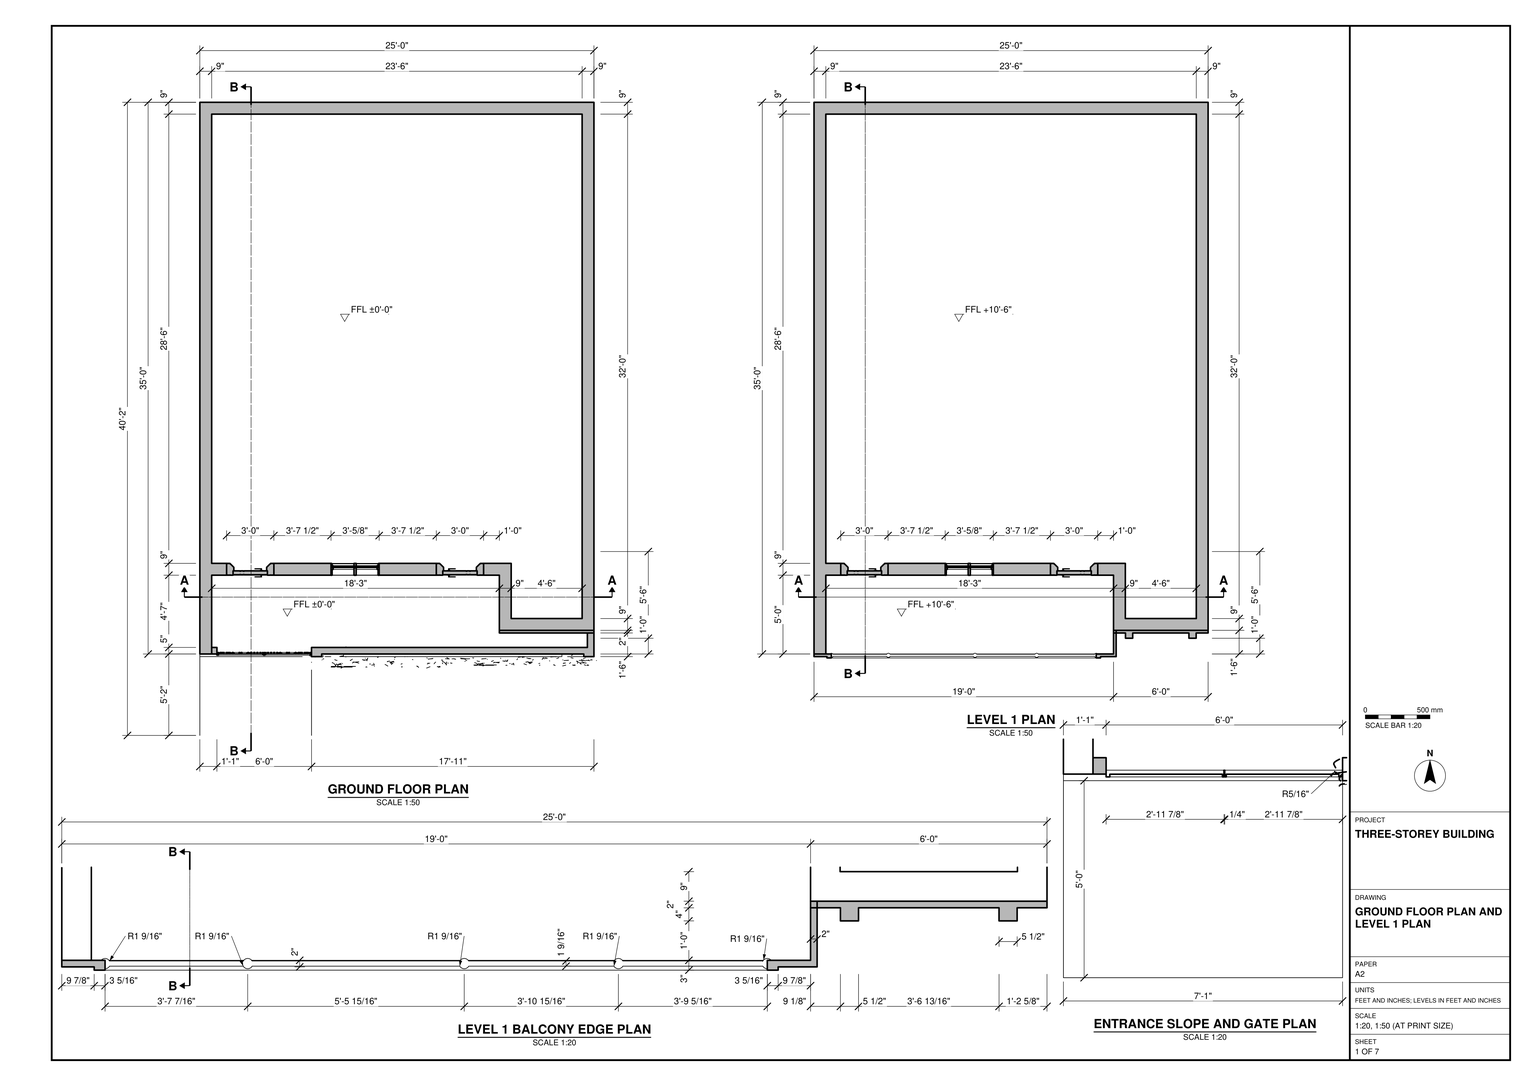
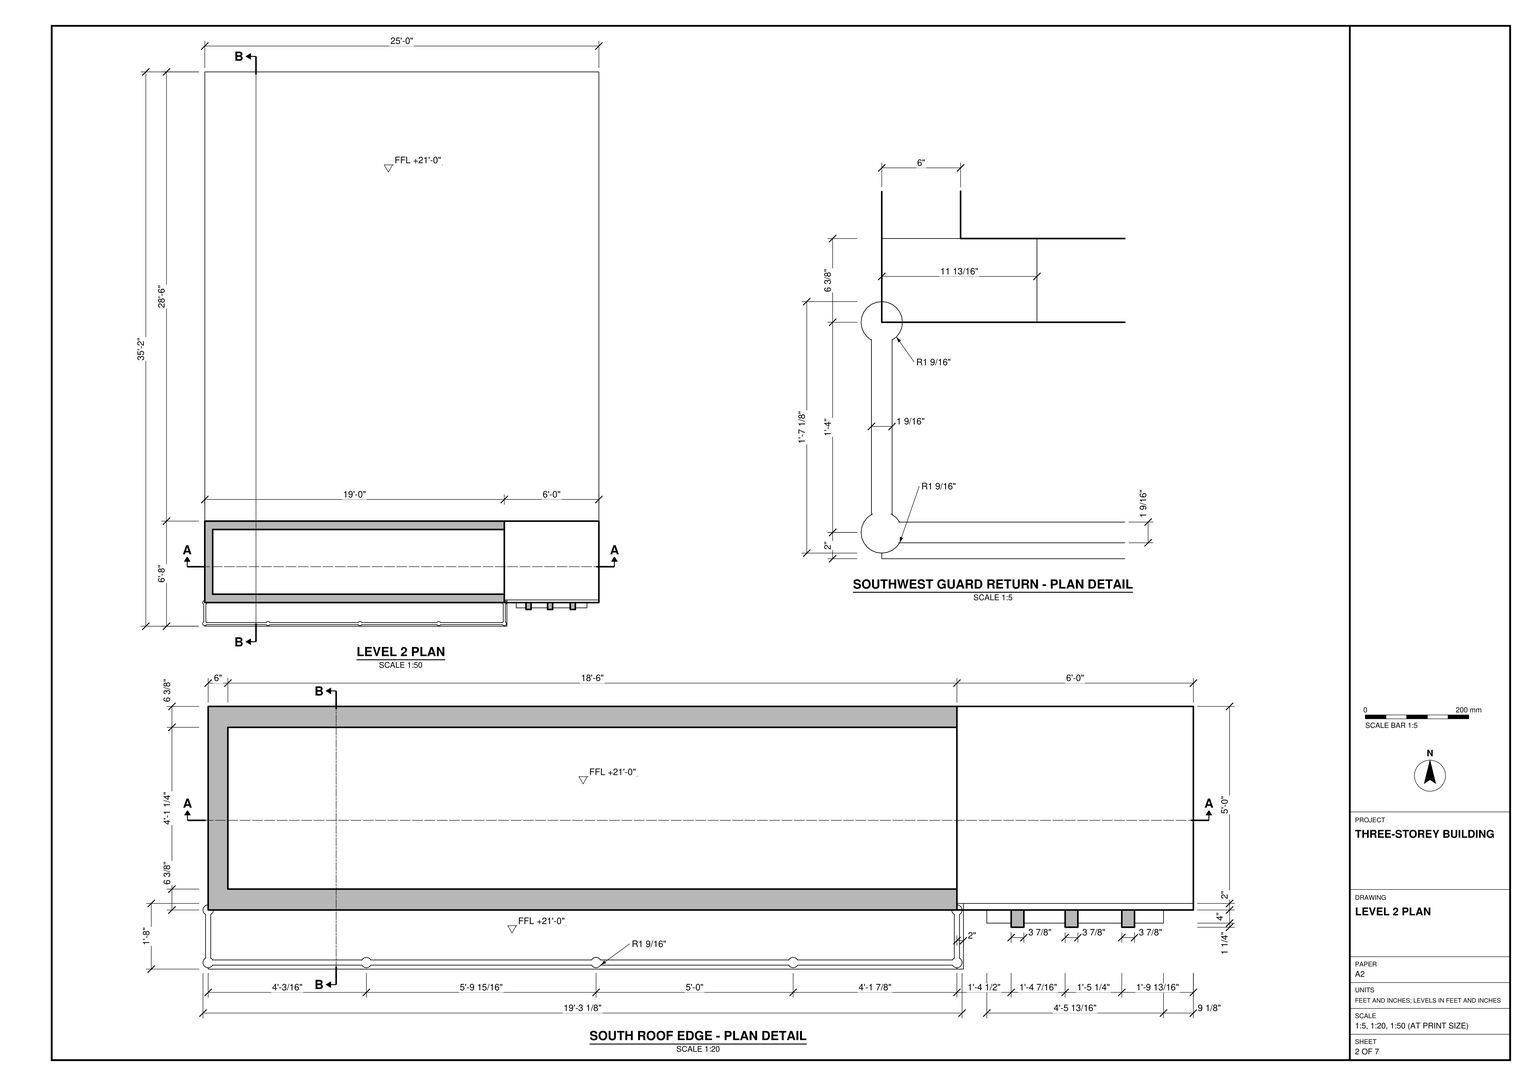
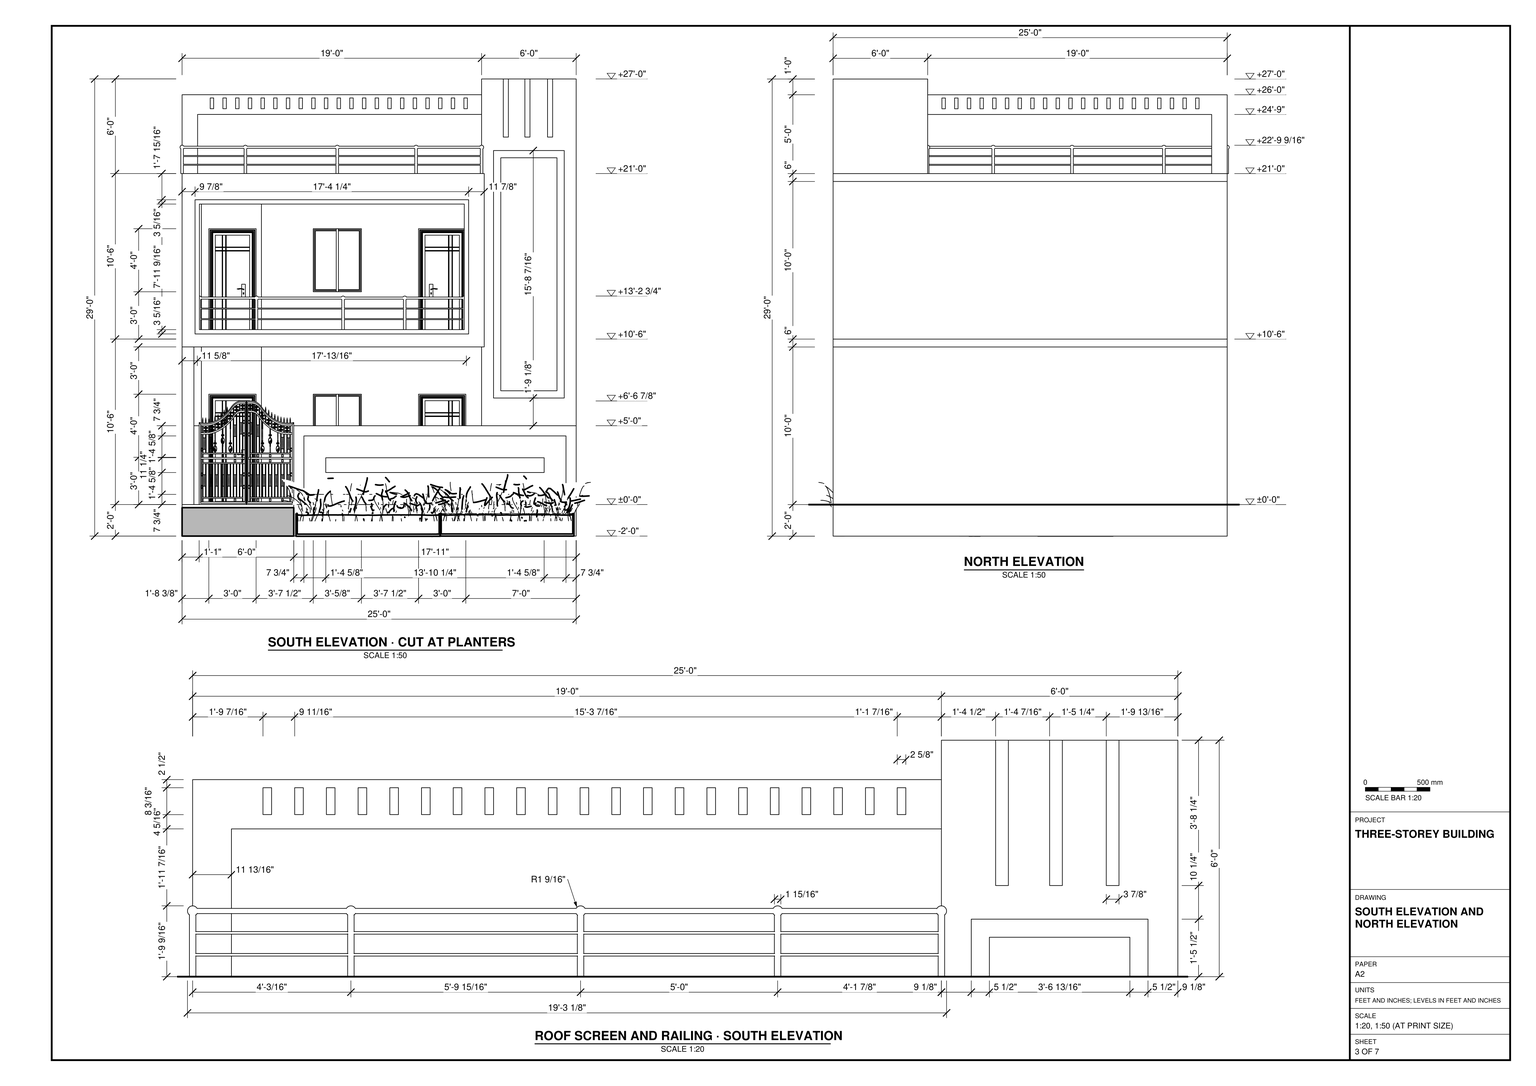
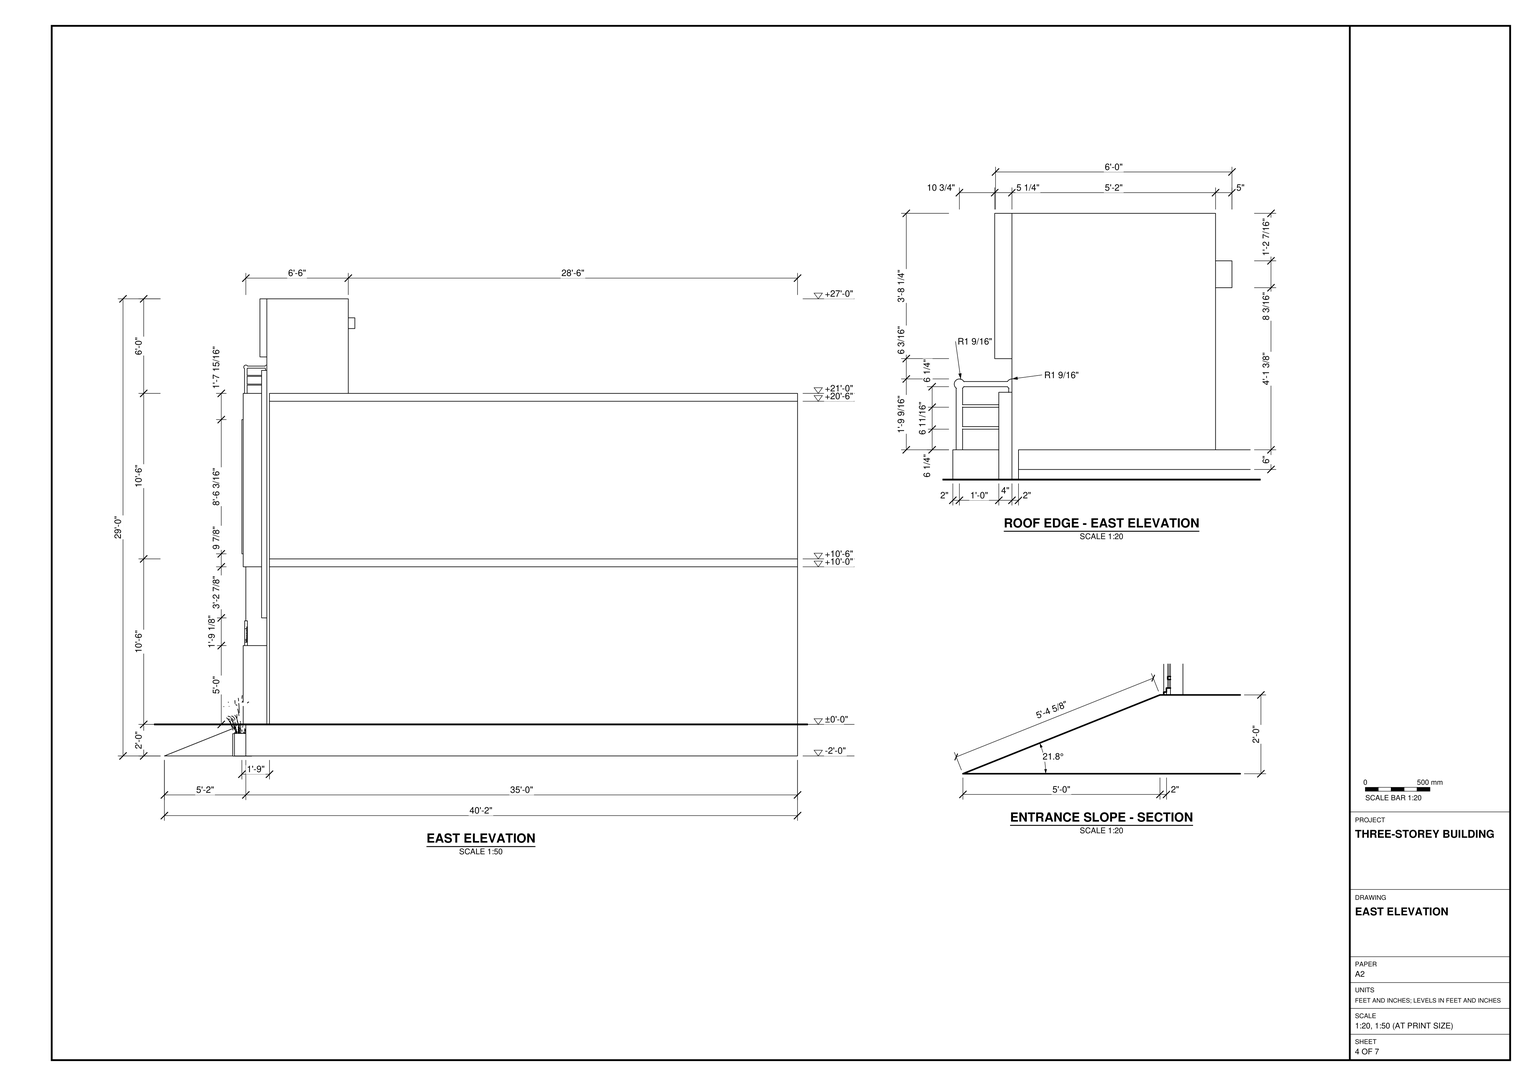
Build the three-storey building in SketchUp from task_files/diagram_01.pdf. Work in feet and inches. Set the overall model extents to 26'-1 5/8" across the frontage, 40'-2" from front to back, and 29'-1/8" from the lowest to the highest point. Use finished levels of ±0'-0" at the ground floor, +10'-6" at the balcony floor, and +21'-0" at the roof terrace.

Lay out the 25'-0" wide shell with the wall thicknesses and stepped south frontage shown in plan. Model the base, floor slabs and flat roof. On the south side, set the doors and central window back from the balcony edge, following the same opening pattern on the ground floor. Frame the balcony opening and distinguish the wide balcony bay from the narrow, taller bay beside it. Use the enlarged details for the balcony guard, roof-edge guard and its returns, slotted roof screen, and vertical strips on the tall bay. At the ground-floor entrance, include the sloping approach, double gate, low wall and planted strip in their drawn positions. Decor and loose items, including plants, may be any suitable library components.

Keep shell elements such as walls, slabs and roof in separate groups or components, and keep each furniture or joinery piece shown separate from the shell. Use components for repeated parts. Save one SketchUp model as output_files/three_storey_building_with_a_balcony_and_roof_screen.skp.

# SketchUp Ruby script. Lengths in inches.
U = 1.inch
M = Sketchup.active_model
def pt(a) = Geom::Point3d.new(a.map { |v| v * U })
def face(e, loops, mat)
  f = e.add_face(loops[0].map { |a| pt(a) })
  loops[1..].each { |l| e.add_face(l.map { |a| pt(a) }).erase! }
  f.material = f.back_material = mat if mat
  f
end
# faces: each face lists its corners as indices into pts; further lists are holes
def faces(e, pts, list, mat = nil) = list.each { |f| face(e, (f[0].is_a?(Array) ? f : [f]).map { |l| l.map { |i| pts[i] } }, mat) }
# xy, xz, yz: faces in a plane at the given z, y or x. An outline is a flat list of corners, or four numbers for a rectangle; further outlines are holes
def ring(l) = l.size == 4 ? [[l[0], l[1]], [l[2], l[1]], [l[2], l[3]], [l[0], l[3]]] : l.each_slice(2).to_a
def flat(e, list, mat, &to3) = list.each { |f| face(e, (f[0].is_a?(Array) ? f : [f]).map { |l| ring(l).map { |u, v| to3.(u, v) } }, mat) }
def xy(e, z, list, mat = nil) = flat(e, list, mat) { |x, y| [x, y, z] }
def xz(e, y, list, mat = nil) = flat(e, list, mat) { |x, z| [x, y, z] }
def yz(e, x, list, mat = nil) = flat(e, list, mat) { |y, z| [x, y, z] }
def lines(e, pts, list) = list.each { |a, b| e.add_line(pt(pts[a]), pt(pts[b])) }
# prism: a flat outline (further loops are holes) pulled along v
def prism(e, loops, v, mat = nil)
  f = face(e, loops, mat); d = Geom::Vector3d.new(v.map { |x| x * U })
  f.pushpull(f.normal.samedirection?(d) ? d.length : -d.length)
end
def box(e, o, s, mat = nil) = prism(e, [[o, [o[0] + s[0], o[1], o[2]], [o[0] + s[0], o[1] + s[1], o[2]], [o[0], o[1] + s[1], o[2]]]], [0, 0, s[2]], mat)
def at(x, y, z, deg = 0) = Geom::Transformation.translation(pt([x, y, z])) * Geom::Transformation.rotation(ORIGIN, Z_AXIS, deg.degrees)
def axes(o, x, y, z) = Geom::Transformation.new([*x, 0, *y, 0, *z, 0, *pt(o).to_a, 1])
def part(name) = M.definitions.add(name)
# library, detail: a bought-in or finely detailed component or shape, given as its bounding box
def library(name, o, s) = part(name).tap { |d| box(d.entities, o, s) }
def detail(e, o, s) = box(e.add_group.entities, o, s)
def put(e, d, t, mat = nil) = e.add_instance(d, t).tap { |i| i.material = mat if mat }
def group(e, t, mat = nil) = e.add_group.tap { |g| g.transformation = t; g.material = mat if mat }.entities
root = M.entities
M.materials.add("[Color A02]").color = [255, 153, 153]
M.materials.add("[Color A07]").color = [153, 0, 0]
M.materials.add("[Color C02]").color = [255, 204, 153]
M.materials.add("[Color I02]").color = [153, 153, 255]
M.materials.add("[Color M02]").color = [198, 198, 198]
M.materials.add("[Color M03]").color = [170, 170, 170]
M.materials.add("[Field Rectangle Tile]").color = [196, 189, 179]
M.materials.add("[Metal Silver]").color = [234, 233, 238]
M.materials.add("[Mirror 01]").color = [185, 185, 185]
M.materials.add("[Tile Hexagon White]").color = [213, 206, 204]
M.materials.add("[Translucent Glass Blue]").color = [100, 149, 237]
M.materials["[Translucent Glass Blue]"].alpha = 0.5
M.materials.add("[Wood Floor Dark]").color = [153, 94, 42]
M.materials.add("white").color = [255, 255, 255]
c1 = part("Support post")
box(c1.entities,[2,0,0],[3.875,5.25,44.25])
c2 = part("Horizontal screen slat")
box(c2.entities,[0,0,0],[2.625,72,8.1875])
c3 = library("bilal architect uae abu dhabi",[0,0,0],[141.6,2.42,96])
c4 = library("House+plant_11",[9.78,20.5,6.2],[56.8,25.91,35.15])
c5 = library("Group\#16",[0,0,0],[36,10.47,84])
c6 = library("Group\#18",[0,0,0],[36,10.47,84])
c7 = part("Group12\#2")
box(c7.entities,[1.02,2.16,1.02],[34.6,0.63,45.96],"[Mirror 01]")
c8 = library("Group\#2",[0,0,0],[36,10.47,84])
c9 = part("Group12\#1")
box(c9.entities,[1.02,2.16,1.02],[34.6,0.63,45.96],"[Mirror 01]")
c10 = library("Group\#1",[0,0,0],[36,10.47,84])
c11 = part("Group\#6")
prism(c11.entities,[[[300,420,0],[300,18,0],[228,18,0],[228,0,0],[0,0,0],[0,420,0]]],[0,0,6])
c12 = library("Ploe",[-1.57,14.43,252],[3.14,3.14,21.57])
c13 = part("Group24\#1")
put(c13.entities,c12,at(0,0,0))
put(c13.entities,c12,at(0,-16,0))
put(c13.entities,c12,at(48.1875,-16,0))
put(c13.entities,c12,at(118.125,-16,0))
put(c13.entities,c12,at(178.125,-16,0))
put(c13.entities,c12,at(228,-16,0))
put(c13.entities,c12,at(228,0,0))
c14 = library("Group25\#1",[-0.79,-0.79,258.27],[229.58,16.79,14.52])
c15 = library("Ploe\#1",[11.6,-2.57,133.17],[3.15,3.14,25.58])
c16 = part("Group28\#1")
put(c16.entities,c15,at(0,0,0))
put(c16.entities,c15,at(43.4375,0,0))
put(c16.entities,c15,at(109.375,0,0))
put(c16.entities,c15,at(156.3125,0,0))
put(c16.entities,c15,at(201.65,0,0))
c17 = part("Group29\#1")
yz(c17.entities,13.17,[[-1,140.78,-1.1,140.79,-1.2,140.83,-1.28,140.9,-1.34,140.98,-1.38,141.07,-1.39,141.17,-1.38,141.28,-1.34,141.37,-1.28,141.45,-1.2,141.51,-1.1,141.55,-1,141.57,-0.9,141.55,-0.8,141.51,-0.72,141.45,-0.66,141.37,-0.62,141.28,-0.61,141.17,-0.62,141.07,-0.66,140.98,-0.72,140.9,-0.8,140.83,-0.9,140.79],[-1,148.78,-1.1,148.79,-1.2,148.83,-1.28,148.9,-1.34,148.98,-1.38,149.07,-1.39,149.17,-1.38,149.28,-1.34,149.37,-1.28,149.45,-1.2,149.51,-1.1,149.55,-1,149.57,-0.9,149.55,-0.8,149.51,-0.72,149.45,-0.66,149.37,-0.62,149.28,-0.61,149.17,-0.62,149.07,-0.66,148.98,-0.72,148.9,-0.8,148.83,-0.9,148.79],[-1,156.39,-1.2,156.41,-1.39,156.49,-1.56,156.62,-1.68,156.78,-1.76,156.97,-1.79,157.17,-1.76,157.38,-1.68,157.57,-1.56,157.73,-1.39,157.86,-1.2,157.93,-1,157.96,-0.8,157.93,-0.61,157.86,-0.44,157.73,-0.32,157.57,-0.24,157.38,-0.21,157.17,-0.24,156.97,-0.32,156.78,-0.44,156.62,-0.61,156.49,-0.8,156.41]])
yz(c17.entities,214.83,[[-1,140.78,-0.9,140.79,-0.8,140.83,-0.72,140.9,-0.66,140.98,-0.62,141.07,-0.61,141.17,-0.62,141.28,-0.66,141.37,-0.72,141.45,-0.8,141.51,-0.9,141.55,-1,141.57,-1.1,141.55,-1.2,141.51,-1.28,141.45,-1.34,141.37,-1.38,141.28,-1.39,141.17,-1.38,141.07,-1.34,140.98,-1.28,140.9,-1.2,140.83,-1.1,140.79],[-1,148.78,-0.9,148.79,-0.8,148.83,-0.72,148.9,-0.66,148.98,-0.62,149.07,-0.61,149.17,-0.62,149.28,-0.66,149.37,-0.72,149.45,-0.8,149.51,-0.9,149.55,-1,149.57,-1.1,149.55,-1.2,149.51,-1.28,149.45,-1.34,149.37,-1.38,149.28,-1.39,149.17,-1.38,149.07,-1.34,148.98,-1.28,148.9,-1.2,148.83,-1.1,148.79],[-1,156.39,-0.8,156.41,-0.61,156.49,-0.44,156.62,-0.32,156.78,-0.24,156.97,-0.21,157.17,-0.24,157.38,-0.32,157.57,-0.44,157.73,-0.61,157.86,-0.8,157.93,-1,157.96,-1.2,157.93,-1.39,157.86,-1.56,157.73,-1.68,157.57,-1.76,157.38,-1.79,157.17,-1.76,156.97,-1.68,156.78,-1.56,156.62,-1.39,156.49,-1.2,156.41]])
p = [[169.49,-1.2,140.83],[214.83,-1.2,140.83],[214.83,-1.28,140.9],[169.49,-1.28,140.9],[122.55,-1.28,140.9],[56.61,-1.28,140.9],
  [13.17,-1.28,140.9],[13.17,-1.2,140.83],[56.61,-1.2,140.83],[122.55,-1.2,140.83],[169.49,-1.1,140.79],[214.83,-1.1,140.79],
  [13.17,-1.1,140.79],[56.61,-1.1,140.79],[122.55,-1.1,140.79],[169.49,-1,140.78],[214.83,-1,140.78],[13.17,-1,140.78],
  [56.61,-1,140.78],[122.55,-1,140.78],[13.17,-0.9,140.79],[56.61,-0.9,140.79],[122.55,-0.9,140.79],[169.49,-0.9,140.79],
  [214.83,-0.9,140.79],[169.49,-0.8,140.83],[214.83,-0.8,140.83],[13.17,-0.8,140.83],[56.61,-0.8,140.83],[122.55,-0.8,140.83],
  [169.49,-0.72,140.9],[214.83,-0.72,140.9],[13.17,-0.72,140.9],[56.61,-0.72,140.9],[122.55,-0.72,140.9],[214.83,-1.34,140.98],
  [169.49,-1.34,140.98],[122.55,-1.34,140.98],[56.61,-1.34,140.98],[13.17,-1.34,140.98],[169.49,-0.66,140.98],[214.83,-0.66,140.98],
  [13.17,-0.66,140.98],[56.61,-0.66,140.98],[122.55,-0.66,140.98],[214.83,-1.38,141.07],[169.49,-1.38,141.07],[122.55,-1.38,141.07],
  [56.61,-1.38,141.07],[13.17,-1.38,141.07],[13.17,-0.62,141.07],[56.61,-0.62,141.07],[122.55,-0.62,141.07],[169.49,-0.62,141.07],
  [214.83,-0.62,141.07],[214.83,-1.39,141.17],[169.49,-1.39,141.17],[122.55,-1.39,141.17],[56.61,-1.39,141.17],[13.17,-1.39,141.17],
  [13.17,-0.61,141.17],[56.61,-0.61,141.17],[122.55,-0.61,141.17],[169.49,-0.61,141.17],[214.83,-0.61,141.17],[214.83,-1.38,141.28],
  [169.49,-1.38,141.28],[122.55,-1.38,141.28],[56.61,-1.38,141.28],[13.17,-1.38,141.28],[13.17,-0.62,141.28],[56.61,-0.62,141.28],
  [122.55,-0.62,141.28],[169.49,-0.62,141.28],[214.83,-0.62,141.28],[214.83,-1.34,141.37],[169.49,-1.34,141.37],[122.55,-1.34,141.37],
  [56.61,-1.34,141.37],[13.17,-1.34,141.37],[56.61,-0.66,141.37],[122.55,-0.66,141.37],[169.49,-0.66,141.37],[214.83,-0.66,141.37],
  [13.17,-0.66,141.37],[214.83,-1.28,141.45],[169.49,-1.28,141.45],[122.55,-1.28,141.45],[56.61,-1.28,141.45],[13.17,-1.28,141.45],
  [13.17,-0.72,141.45],[56.61,-0.72,141.45],[122.55,-0.72,141.45],[169.49,-0.72,141.45],[214.83,-0.72,141.45],[214.83,-1.2,141.51],
  [169.49,-1.2,141.51],[122.55,-1.2,141.51],[56.61,-1.2,141.51],[13.17,-1.2,141.51],[214.83,-1.1,141.55],[169.49,-1.1,141.55],
  [122.55,-1.1,141.55],[56.61,-1.1,141.55],[13.17,-1.1,141.55],[56.61,-0.9,141.55],[122.55,-0.9,141.55],[169.49,-0.9,141.55],
  [214.83,-0.9,141.55],[214.83,-0.8,141.51],[169.49,-0.8,141.51],[122.55,-0.8,141.51],[56.61,-0.8,141.51],[13.17,-0.8,141.51],
  [13.17,-0.9,141.55],[13.17,-1,141.57],[214.83,-1,141.57],[169.49,-1,141.57],[122.55,-1,141.57],[56.61,-1,141.57],
  [56.61,-1.2,148.83],[122.55,-1.2,148.83],[169.49,-1.2,148.83],[214.83,-1.2,148.83],[214.83,-1.28,148.9],[169.49,-1.28,148.9],
  [122.55,-1.28,148.9],[56.61,-1.28,148.9],[13.17,-1.28,148.9],[13.17,-1.2,148.83],[13.17,-1.1,148.79],[56.61,-1.1,148.79],
  [122.55,-1.1,148.79],[169.49,-1.1,148.79],[214.83,-1.1,148.79],[56.61,-1,148.78],[122.55,-1,148.78],[169.49,-1,148.78],
  [214.83,-1,148.78],[13.17,-1,148.78],[169.49,-0.9,148.79],[214.83,-0.9,148.79],[13.17,-0.9,148.79],[56.61,-0.9,148.79],
  [122.55,-0.9,148.79],[13.17,-0.8,148.83],[56.61,-0.8,148.83],[122.55,-0.8,148.83],[169.49,-0.8,148.83],[214.83,-0.8,148.83],
  [169.49,-0.72,148.9],[214.83,-0.72,148.9],[13.17,-0.72,148.9],[56.61,-0.72,148.9],[122.55,-0.72,148.9],[214.83,-1.34,148.98],
  [169.49,-1.34,148.98],[122.55,-1.34,148.98],[56.61,-1.34,148.98],[13.17,-1.34,148.98],[169.49,-0.66,148.98],[214.83,-0.66,148.98],
  [13.17,-0.66,148.98],[56.61,-0.66,148.98],[122.55,-0.66,148.98],[13.17,-1.38,149.07],[214.83,-1.38,149.07],[169.49,-1.38,149.07],
  [122.55,-1.38,149.07],[56.61,-1.38,149.07],[169.49,-0.62,149.07],[214.83,-0.62,149.07],[13.17,-0.62,149.07],[56.61,-0.62,149.07],
  [122.55,-0.62,149.07],[214.83,-1.39,149.17],[169.49,-1.39,149.17],[122.55,-1.39,149.17],[56.61,-1.39,149.17],[13.17,-1.39,149.17],
  [13.17,-0.61,149.17],[56.61,-0.61,149.17],[122.55,-0.61,149.17],[169.49,-0.61,149.17],[214.83,-0.61,149.17],[13.17,-1.38,149.28],
  [214.83,-1.38,149.28],[169.49,-1.38,149.28],[122.55,-1.38,149.28],[56.61,-1.38,149.28],[13.17,-0.62,149.28],[56.61,-0.62,149.28],
  [122.55,-0.62,149.28],[169.49,-0.62,149.28],[214.83,-0.62,149.28],[214.83,-1.34,149.37],[169.49,-1.34,149.37],[122.55,-1.34,149.37],
  [56.61,-1.34,149.37],[13.17,-1.34,149.37],[13.17,-0.66,149.37],[56.61,-0.66,149.37],[122.55,-0.66,149.37],[169.49,-0.66,149.37],
  [214.83,-0.66,149.37],[13.17,-1.28,149.45],[214.83,-1.28,149.45],[169.49,-1.28,149.45],[122.55,-1.28,149.45],[56.61,-1.28,149.45],
  [56.61,-0.72,149.45],[122.55,-0.72,149.45],[169.49,-0.72,149.45],[214.83,-0.72,149.45],[13.17,-0.72,149.45],[13.17,-1.2,149.51],
  [214.83,-1.2,149.51],[169.49,-1.2,149.51],[122.55,-1.2,149.51],[56.61,-1.2,149.51],[13.17,-1.1,149.55],[214.83,-1.1,149.55],
  [169.49,-1.1,149.55],[122.55,-1.1,149.55],[56.61,-1.1,149.55],[56.61,-0.9,149.55],[122.55,-0.9,149.55],[169.49,-0.9,149.55],
  [214.83,-0.9,149.55],[214.83,-0.8,149.51],[169.49,-0.8,149.51],[122.55,-0.8,149.51],[56.61,-0.8,149.51],[13.17,-0.8,149.51],
  [13.17,-0.9,149.55],[13.17,-1,149.57],[214.83,-1,149.57],[169.49,-1,149.57],[122.55,-1,149.57],[56.61,-1,149.57],
  [13.17,-1.39,156.49],[13.17,-1.2,156.41],[56.61,-1.2,156.41],[122.55,-1.2,156.41],[169.49,-1.2,156.41],[214.83,-1.2,156.41],
  [214.83,-1.39,156.49],[169.49,-1.39,156.49],[122.55,-1.39,156.49],[56.61,-1.39,156.49],[13.17,-1,156.39],[56.61,-1,156.39],
  [122.55,-1,156.39],[169.49,-1,156.39],[214.83,-1,156.39],[13.17,-0.8,156.41],[56.61,-0.8,156.41],[122.55,-0.8,156.41],
  [169.49,-0.8,156.41],[214.83,-0.8,156.41],[169.49,-0.61,156.49],[214.83,-0.61,156.49],[13.17,-0.61,156.49],[56.61,-0.61,156.49],
  [122.55,-0.61,156.49],[214.83,-1.56,156.62],[169.49,-1.56,156.62],[122.55,-1.56,156.62],[56.61,-1.56,156.62],[13.17,-1.56,156.62],
  [56.61,-0.44,156.62],[122.55,-0.44,156.62],[169.49,-0.44,156.62],[214.83,-0.44,156.62],[13.17,-0.44,156.62],[214.83,-1.68,156.78],
  [169.49,-1.68,156.78],[122.55,-1.68,156.78],[56.61,-1.68,156.78],[13.17,-1.68,156.78],[13.17,-0.32,156.78],[56.61,-0.32,156.78],
  [122.55,-0.32,156.78],[169.49,-0.32,156.78],[214.83,-0.32,156.78],[214.83,-1.76,156.97],[169.49,-1.76,156.97],[122.55,-1.76,156.97],
  [56.61,-1.76,156.97],[13.17,-1.76,156.97],[13.17,-0.24,156.97],[56.61,-0.24,156.97],[122.55,-0.24,156.97],[169.49,-0.24,156.97],
  [214.83,-0.24,156.97],[214.83,-1.79,157.17],[169.49,-1.79,157.17],[122.55,-1.79,157.17],[56.61,-1.79,157.17],[13.17,-1.79,157.17],
  [13.17,-0.21,157.17],[56.61,-0.21,157.17],[122.55,-0.21,157.17],[169.49,-0.21,157.17],[214.83,-0.21,157.17],[214.83,-1.76,157.38],
  [169.49,-1.76,157.38],[122.55,-1.76,157.38],[56.61,-1.76,157.38],[13.17,-1.76,157.38],[169.49,-0.24,157.38],[214.83,-0.24,157.38],
  [13.17,-0.24,157.38],[56.61,-0.24,157.38],[122.55,-0.24,157.38],[214.83,-1.68,157.57],[169.49,-1.68,157.57],[122.55,-1.68,157.57],
  [56.61,-1.68,157.57],[13.17,-1.68,157.57],[13.17,-0.32,157.57],[56.61,-0.32,157.57],[122.55,-0.32,157.57],[169.49,-0.32,157.57],
  [214.83,-0.32,157.57],[13.17,-1.56,157.73],[214.83,-1.56,157.73],[169.49,-1.56,157.73],[122.55,-1.56,157.73],[56.61,-1.56,157.73],
  [13.17,-0.44,157.73],[56.61,-0.44,157.73],[122.55,-0.44,157.73],[169.49,-0.44,157.73],[214.83,-0.44,157.73],[214.83,-1.39,157.86],
  [169.49,-1.39,157.86],[122.55,-1.39,157.86],[56.61,-1.39,157.86],[13.17,-1.39,157.86],[13.17,-0.61,157.86],[56.61,-0.61,157.86],
  [122.55,-0.61,157.86],[169.49,-0.61,157.86],[214.83,-0.61,157.86],[214.83,-1.2,157.93],[169.49,-1.2,157.93],[122.55,-1.2,157.93],
  [56.61,-1.2,157.93],[13.17,-1.2,157.93],[214.83,-1,157.96],[169.49,-1,157.96],[122.55,-1,157.96],[56.61,-1,157.96],
  [13.17,-1,157.96],[13.17,-0.8,157.93],[214.83,-0.8,157.93],[169.49,-0.8,157.93],[122.55,-0.8,157.93],[56.61,-0.8,157.93]]
faces(c17.entities,p,[[0,1,2,3,4,5,6,7,8,9],[10,11,1,0,9,8,7,12,13,14],[15,16,11,10,14,13,12,17,18,19],[17,20,21,22,23,24,16,15,19,18],[25,26,24,23,22,21,20,27,28,29],[30,31,26,25,29,28,27,32,33,34],[5,4,3,2,35,36,37,38,39,6],[40,41,31,30,34,33,32,42,43,44],
  [38,37,36,35,45,46,47,48,49,39],[42,50,51,52,53,54,41,40,44,43],[46,45,55,56,57,58,59,49,48,47],[50,60,61,62,63,64,54,53,52,51],[58,57,56,55,65,66,67,68,69,59],[60,70,71,72,73,74,64,63,62,61],[68,67,66,65,75,76,77,78,79,69],[80,81,82,83,74,73,72,71,70,84],
  [78,77,76,75,85,86,87,88,89,79],[84,90,91,92,93,94,83,82,81,80],[88,87,86,85,95,96,97,98,99,89],[98,97,96,95,100,101,102,103,104,99],[105,106,107,108,109,110,111,112,113,114],[90,113,112,111,110,109,94,93,92,91],[115,104,103,102,101,100,116,117,118,119],[114,115,119,118,117,116,108,107,106,105],
  [120,121,122,123,124,125,126,127,128,129],[129,130,131,132,133,134,123,122,121,120],[135,136,137,138,134,133,132,131,130,139],[140,141,138,137,136,135,139,142,143,144],[142,145,146,147,148,149,141,140,144,143],[150,151,149,148,147,146,145,152,153,154],[125,124,155,156,157,158,159,128,127,126],[160,161,151,150,154,153,152,162,163,164],
  [165,159,158,157,156,155,166,167,168,169],[170,171,161,160,164,163,162,172,173,174],[169,168,167,166,175,176,177,178,179,165],[172,180,181,182,183,184,171,170,174,173],[185,179,178,177,176,175,186,187,188,189],[180,190,191,192,193,194,184,183,182,181],[189,188,187,186,195,196,197,198,199,185],[190,200,201,202,203,204,194,193,192,191],
  [205,199,198,197,196,195,206,207,208,209],[210,211,212,213,204,203,202,201,200,214],[215,205,209,208,207,206,216,217,218,219],[220,215,219,218,217,216,221,222,223,224],[225,226,227,228,229,230,231,232,233,234],[232,231,230,229,213,212,211,210,214,233],[235,220,224,223,222,221,236,237,238,239],[234,235,239,238,237,236,228,227,226,225],
  [240,241,242,243,244,245,246,247,248,249],[241,250,251,252,253,254,245,244,243,242],[250,255,256,257,258,259,254,253,252,251],[260,261,259,258,257,256,255,262,263,264],[249,248,247,246,265,266,267,268,269,240],[270,271,272,273,261,260,264,263,262,274],[266,265,275,276,277,278,279,269,268,267],[274,280,281,282,283,284,273,272,271,270],
  [276,275,285,286,287,288,289,279,278,277],[280,290,291,292,293,294,284,283,282,281],[286,285,295,296,297,298,299,289,288,287],[290,300,301,302,303,304,294,293,292,291],[298,297,296,295,305,306,307,308,309,299],[310,311,304,303,302,301,300,312,313,314],[308,307,306,305,315,316,317,318,319,309],[312,320,321,322,323,324,311,310,314,313],
  [325,319,318,317,316,315,326,327,328,329],[320,330,331,332,333,334,324,323,322,321],[329,328,327,326,335,336,337,338,339,325],[330,340,341,342,343,344,334,333,332,331],[338,337,336,335,345,346,347,348,349,339],[348,347,346,345,350,351,352,353,354,349],[355,354,353,352,351,350,356,357,358,359],[359,358,357,356,344,343,342,341,340,355]])
p = [[13.17,60,133.17],[214.83,60,133.17]]
lines(root,p,[[0,1]])
put(root,c1,at(242.52,72.75,279.75))
put(root,c1,at(258.95,72.75,279.75))
put(root,c1,at(276.2,72.75,279.75))
put(root,c2,at(21.42,73,301.35),"[Color A07]")
put(root,c2,at(31.07,73,301.35),"[Color A07]")
put(root,c2,at(40.73,73,301.35),"[Color A07]")
put(root,c2,at(50.38,73,301.35),"[Color A07]")
put(root,c2,at(60.04,73,301.35),"[Color A07]")
put(root,c2,at(69.7,73,301.35),"[Color A07]")
put(root,c2,at(79.35,73,301.35),"[Color A07]")
put(root,c2,at(89.01,73,301.35),"[Color A07]")
put(root,c2,at(98.67,73,301.35),"[Color A07]")
put(root,c2,at(108.32,73,301.35),"[Color A07]")
put(root,c2,at(117.98,73,301.35),"[Color A07]")
put(root,c2,at(127.63,73,301.35),"[Color A07]")
put(root,c2,at(137.29,73,301.35),"[Color A07]")
put(root,c2,at(146.95,73,301.35),"[Color A07]")
put(root,c2,at(156.6,73,301.35),"[Color A07]")
put(root,c2,at(166.26,73,301.35),"[Color A07]")
put(root,c2,at(175.92,73,301.35),"[Color A07]")
put(root,c2,at(185.57,73,301.35),"[Color A07]")
put(root,c2,at(195.23,73,301.35),"[Color A07]")
put(root,c2,at(204.88,73,301.35),"[Color A07]")
put(root,c2,at(214.54,73,301.35),"[Color A07]")
put(root,c3,axes([13,61.15,0],[0.50848,0,0],[0,0.84384,0],[0,0,0.8215]))
put(root,c4,axes([160.875,34.89,-32.45],[2.27085,0,0],[0,0.68115,0],[0,0,1.36]))
put(root,c4,axes([48.88,21.13,-32.59],[2.43767,0,0],[0,1.14003,0],[0,0,1.36]))
put(root,c5,at(20.35,120.53,0),"[Color C02]")
put(root,c6,at(180,120.53,0))
g1 = group(root,at(136.5,131,36,180))
g2 = group(g1,at(0,0,0),"[Metal Silver]")
xy(g2,0,[[0,0,17.5,9],[17.5,0,19.15,9],[19.15,0,36.65,9]])
xy(g2,0.83,[[0.83,4.61,17.5,8.93],[19.15,4.61,35.82,8.93]])
xy(g2,1.02,[[1.02,2.16,17.5,3.3125],[17.5,2.16,19.15,3.3125],[19.15,2.16,35.62,3.3125]])
xy(g2,1.61,[[1.61,1.8,17.5,2.16],[19.15,1.8,35.03,2.16]])
xy(g2,1.65,[[1.65,3.3125,17.5,3.46],[19.15,3.3125,34.99,3.46]])
xy(g2,46.35,[[1.65,3.3125,17.5,3.46],[19.15,3.3125,34.99,3.46]])
xy(g2,46.39,[[1.61,1.8,17.5,2.16],[19.15,1.8,35.03,2.16]])
xy(g2,46.98,[[1.02,2.16,17.5,3.3125],[17.5,2.16,19.15,3.3125],[19.15,2.16,35.62,3.3125]])
xy(g2,47.17,[[0.83,4.61,17.5,8.93],[19.15,4.61,35.82,8.93]])
xy(g2,48,[[0,0,17.5,9],[17.5,0,19.15,9],[19.15,0,36.65,9]])
xz(g2,0,[[0,0,17.5,0,17.5,0.39,0.39,0.39,0.39,47.61,17.5,47.61,17.5,48,0,48],[17.5,0,19.15,48],[19.15,0,36.65,0,36.65,48,19.15,48,19.15,47.61,36.25,47.61,36.25,0.39,19.15,0.39]])
xz(g2,0.36,[[0.59,0.59,17.5,0.59,17.5,0.79,0.79,0.79,0.79,47.21,17.5,47.21,17.5,47.41,0.59,47.41],[19.15,0.59,36.06,0.59,36.06,47.41,19.15,47.41,19.15,47.21,35.86,47.21,35.86,0.79,19.15,0.79]])
xz(g2,1.8,[[0.83,0.83,17.5,0.83,17.5,1.61,1.61,1.61,1.61,46.39,17.5,46.39,17.5,47.17,0.83,47.17],[19.15,0.83,35.82,0.83,35.82,47.17,19.15,47.17,19.15,46.39,35.03,46.39,35.03,1.61,19.15,1.61]])
xz(g2,2.16,[[1.02,1.02,1.02,46.98,17.5,46.98,17.5,46.39,1.61,46.39,1.61,1.61,17.5,1.61,17.5,1.02],[17.5,1.02,19.15,46.98],[19.15,1.02,19.15,1.61,35.03,1.61,35.03,46.39,19.15,46.39,19.15,46.98,35.62,46.98,35.62,1.02]])
xz(g2,3.3125,[[1.02,1.02,17.5,1.02,17.5,1.65,1.65,1.65,1.65,46.35,17.5,46.35,17.5,46.98,1.02,46.98],[17.5,1.02,19.15,46.98],[19.15,1.02,35.62,1.02,35.62,46.98,19.15,46.98,19.15,46.35,34.99,46.35,34.99,1.65,19.15,1.65]])
xz(g2,4.61,[[0.83,0.83,0.83,47.17,17.5,47.17,17.5,46.5,1.5,46.5,1.5,1.5,17.5,1.5,17.5,0.83],[19.15,0.83,19.15,1.5,35.15,1.5,35.15,46.5,19.15,46.5,19.15,47.17,35.82,47.17,35.82,0.83]],"[Color M03]")
xz(g2,9.07,[[0.04,0.04,0.04,47.96,17.5,47.96,17.5,47.25,0.75,47.25,0.75,0.75,17.5,0.75,17.5,0.04],[17.5,0.04,19.15,47.96],[19.15,0.04,19.15,0.75,35.9,0.75,35.9,47.25,19.15,47.25,19.15,47.96,36.61,47.96,36.61,0.04]],"[Color M03]")
yz(g2,0,[[0,0,9,48]])
yz(g2,0.83,[[4.61,0.83,8.93,47.17]])
yz(g2,1.02,[[2.16,1.02,3.3125,46.98]])
yz(g2,1.61,[[1.8,1.61,2.16,46.39]])
yz(g2,1.65,[[3.3125,1.65,3.46,46.35]])
yz(g2,17.5,[[0,0,9,0,9.07,0.04,9.07,0.75,8.93,0.83,4.61,0.83,4.61,1.5,3.46,1.65,3.3125,1.65,3.3125,1.02,2.16,1.02,2.16,1.61,1.8,1.61,1.8,0.83,0.36,0.79,0.36,0.59,0,0.39],[3.3125,46.35,3.46,46.35,4.61,46.5,4.61,47.17,8.93,47.17,9.07,47.25,9.07,47.96,9,48,0,48,0,47.61,0.36,47.41,0.36,47.21,1.8,47.17,1.8,46.39,2.16,46.39,2.16,46.98,3.3125,46.98]])
yz(g2,17.5,[[[0,0,0,48,9,48,9.07,47.96,9.07,0.04,9,0],[2.16,1.02,3.3125,46.98]]],"[Color M03]")
yz(g2,19.15,[[0,0,0,0.39,0.36,0.59,0.36,0.79,1.8,0.83,1.8,1.61,2.16,1.61,2.16,1.02,3.3125,1.02,3.3125,1.65,3.46,1.65,4.61,1.5,4.61,0.83,8.93,0.83,9.07,0.75,9.07,0.04,9,0],[[0,0,9,0,9.07,0.04,9.07,47.96,9,48,0,48],[2.16,1.02,3.3125,46.98]],[3.3125,46.35,3.3125,46.98,2.16,46.98,2.16,46.39,1.8,46.39,1.8,47.17,0.36,47.21,0.36,47.41,0,47.61,0,48,9,48,9.07,47.96,9.07,47.25,8.93,47.17,4.61,47.17,4.61,46.5,3.46,46.35]])
yz(g2,34.99,[[3.3125,1.65,3.46,46.35]])
yz(g2,35.03,[[1.8,1.61,2.16,46.39]])
yz(g2,35.62,[[2.16,1.02,3.3125,46.98]])
yz(g2,35.82,[[4.61,0.83,8.93,47.17]])
yz(g2,36.65,[[0,0,9,48]])
p = [[17.5,9.07,0.04],[17.5,9,0],[0,9,0],[0.04,9.07,0.04],[0,9,48],[0.04,9.07,47.96],
  [19.15,9.07,0.04],[19.15,9,0],[36.61,9.07,0.04],[36.65,9,0],[36.61,9.07,47.96],[36.65,9,48],
  [17.5,0,0.39],[17.5,0.36,0.59],[0.59,0.36,0.59],[0.39,0,0.39],[0.59,0.36,47.41],[0.39,0,47.61],
  [19.15,0.36,0.59],[19.15,0,0.39],[36.25,0,0.39],[36.06,0.36,0.59],[36.25,0,47.61],[36.06,0.36,47.41],
  [17.5,8.93,0.83],[17.5,9.07,0.75],[0.75,9.07,0.75],[0.83,8.93,0.83],[0.75,9.07,47.25],[0.83,8.93,47.17],
  [19.15,9.07,0.75],[19.15,8.93,0.83],[35.82,8.93,0.83],[35.9,9.07,0.75],[35.82,8.93,47.17],[35.9,9.07,47.25],
  [17.5,0.36,0.79],[17.5,1.8,0.83],[0.83,1.8,0.83],[0.79,0.36,0.79],[0.83,1.8,47.17],[0.79,0.36,47.21],
  [19.15,1.8,0.83],[19.15,0.36,0.79],[35.86,0.36,0.79],[35.82,1.8,0.83],[35.86,0.36,47.21],[35.82,1.8,47.17],
  [17.5,3.46,1.65],[17.5,4.61,1.5],[1.5,4.61,1.5],[1.65,3.46,1.65],[1.5,4.61,46.5],[1.65,3.46,46.35],
  [19.15,4.61,1.5],[19.15,3.46,1.65],[34.99,3.46,1.65],[35.15,4.61,1.5],[34.99,3.46,46.35],[35.15,4.61,46.5],
  [17.5,4.61,46.5],[17.5,3.46,46.35],[19.15,3.46,46.35],[19.15,4.61,46.5],[17.5,1.8,47.17],[17.5,0.36,47.21],
  [19.15,0.36,47.21],[19.15,1.8,47.17],[17.5,9.07,47.25],[17.5,8.93,47.17],[19.15,8.93,47.17],[19.15,9.07,47.25],
  [17.5,0.36,47.41],[17.5,0,47.61],[19.15,0,47.61],[19.15,0.36,47.41],[17.5,9,48],[17.5,9.07,47.96],
  [19.15,9,48],[19.15,9.07,47.96]]
faces(g2,p,[[0,1,2,3],[3,2,4,5],[1,0,6,7],[7,6,8,9],[9,8,10,11],[12,13,14,15],[15,14,16,17],[18,19,20,21],
  [21,20,22,23],[24,25,26,27],[27,26,28,29],[30,31,32,33],[33,32,34,35],[36,37,38,39],[39,38,40,41],[42,43,44,45],
  [45,44,46,47],[48,49,50,51],[51,50,52,53],[57,56,58,59],[53,52,60,61],[59,58,62,63],[41,40,64,65],[47,46,66,67],
  [29,28,68,69],[35,34,70,71],[17,16,72,73],[23,22,74,75],[5,4,76,77],[77,76,78,79],[11,10,79,78]])
faces(g2,p,[[54,55,56,57]],"[Color M03]")
put(g1,c7,at(0,0,0),"[Translucent Glass Blue]")
g3 = group(root,at(0,62,0))
xy(g3,0,[[0,0,0,420,300,420,300,18,228,18,228,60,216,60,216,69,237,69,237,27,291,27,291,411,9,411,9,69,20.35,69,20.35,60,9,60,9,0],[56.35,60,180,69]])
xy(g3,36,[[99.85,60,136.5,69]])
xy(g3,84,[[20.35,60,56.35,69],[99.85,60,136.5,69],[180,60,216,69]])
xy(g3,120,[[[0,0,9,0,9,60,228,60,228,18,300,18,300,420,0,420],[237,27,237,69,9,69,9,411,291,411,291,27]]])
xz(g3,0,[[0,0,9,120]])
xz(g3,18,[[228,0,300,120]])
xz(g3,27,[[237,0,291,120]])
xz(g3,60,[[9,0,14.68,120],[[60.4,0,180,0,180,84,216,84,216,0,228,0,228,120,60.4,120],[99.85,36,136.5,84]]])
xz(g3,60,[[14.68,0,20.35,0,20.35,84,56.35,84,56.35,0,60.4,0,60.4,120,14.68,120]],"[Wood Floor Dark]")
xz(g3,69,[[[9,0,9,120,237,120,237,0,216,0,216,84,180,84,180,0,56.35,0,56.35,84,20.35,84,20.35,0],[99.85,36,136.5,84]]])
xz(g3,411,[[9,0,291,120]])
xz(g3,420,[[0,0,300,120]])
yz(g3,0,[[0,0,420,120]])
yz(g3,9,[[0,0,60,120],[69,0,411,120]])
yz(g3,20.35,[[60,0,69,84]])
yz(g3,56.35,[[60,0,69,84]])
yz(g3,99.85,[[60,36,69,84]])
yz(g3,136.5,[[60,36,69,84]])
yz(g3,180,[[60,0,69,84]])
yz(g3,216,[[60,0,69,84]])
yz(g3,228,[[18,0,60,120]])
yz(g3,237,[[27,0,69,120]])
yz(g3,291,[[27,0,411,120]])
yz(g3,300,[[18,0,420,120]])
p = [[56.35,60,0],[20.35,60,0]]
lines(g3,p,[[0,1]])
put(root,c8,at(180,120.53,126))
g4 = group(root,at(136.5,131,162,180),"[Color M02]")
g5 = group(g4,at(0,0,0),"[Color M03]")
xy(g5,0,[[0,0,17.5,9],[17.5,0,19.15,9],[19.15,0,36.65,9]])
xy(g5,0.83,[[0.83,4.61,17.5,8.93],[19.15,4.61,35.82,8.93]])
xy(g5,1.02,[[1.02,2.16,17.5,3.3125],[17.5,2.16,19.15,3.3125],[19.15,2.16,35.62,3.3125]])
xy(g5,1.61,[[1.61,1.8,17.5,2.16],[19.15,1.8,35.03,2.16]])
xy(g5,1.65,[[1.65,3.3125,17.5,3.46],[19.15,3.3125,34.99,3.46]])
xy(g5,46.35,[[1.65,3.3125,17.5,3.46],[19.15,3.3125,34.99,3.46]])
xy(g5,46.39,[[1.61,1.8,17.5,2.16],[19.15,1.8,35.03,2.16]])
xy(g5,46.98,[[1.02,2.16,17.5,3.3125],[17.5,2.16,19.15,3.3125],[19.15,2.16,35.62,3.3125]])
xy(g5,47.17,[[0.83,4.61,17.5,8.93],[19.15,4.61,35.82,8.93]])
xy(g5,48,[[0,0,17.5,9],[17.5,0,19.15,9],[19.15,0,36.65,9]])
xz(g5,0,[[0,0,17.5,0,17.5,0.39,0.39,0.39,0.39,47.61,17.5,47.61,17.5,48,0,48],[17.5,0,19.15,48],[19.15,0,36.65,0,36.65,48,19.15,48,19.15,47.61,36.25,47.61,36.25,0.39,19.15,0.39]])
xz(g5,0.36,[[0.59,0.59,17.5,0.59,17.5,0.79,0.79,0.79,0.79,47.21,17.5,47.21,17.5,47.41,0.59,47.41],[19.15,0.59,36.06,0.59,36.06,47.41,19.15,47.41,19.15,47.21,35.86,47.21,35.86,0.79,19.15,0.79]])
xz(g5,1.8,[[0.83,0.83,17.5,0.83,17.5,1.61,1.61,1.61,1.61,46.39,17.5,46.39,17.5,47.17,0.83,47.17],[19.15,0.83,35.82,0.83,35.82,47.17,19.15,47.17,19.15,46.39,35.03,46.39,35.03,1.61,19.15,1.61]])
xz(g5,2.16,[[1.02,1.02,1.02,46.98,17.5,46.98,17.5,46.39,1.61,46.39,1.61,1.61,17.5,1.61,17.5,1.02],[17.5,1.02,19.15,46.98],[19.15,1.02,19.15,1.61,35.03,1.61,35.03,46.39,19.15,46.39,19.15,46.98,35.62,46.98,35.62,1.02]])
xz(g5,3.3125,[[1.02,1.02,17.5,1.02,17.5,1.65,1.65,1.65,1.65,46.35,17.5,46.35,17.5,46.98,1.02,46.98],[17.5,1.02,19.15,46.98],[19.15,1.02,35.62,1.02,35.62,46.98,19.15,46.98,19.15,46.35,34.99,46.35,34.99,1.65,19.15,1.65]])
xz(g5,4.61,[[0.83,0.83,0.83,47.17,17.5,47.17,17.5,46.5,1.5,46.5,1.5,1.5,17.5,1.5,17.5,0.83],[19.15,0.83,19.15,1.5,35.15,1.5,35.15,46.5,19.15,46.5,19.15,47.17,35.82,47.17,35.82,0.83]])
xz(g5,9.07,[[0.04,0.04,0.04,47.96,17.5,47.96,17.5,47.25,0.75,47.25,0.75,0.75,17.5,0.75,17.5,0.04],[17.5,0.04,19.15,47.96],[19.15,0.04,19.15,0.75,35.9,0.75,35.9,47.25,19.15,47.25,19.15,47.96,36.61,47.96,36.61,0.04]])
yz(g5,0,[[0,0,9,48]])
yz(g5,0.83,[[4.61,0.83,8.93,47.17]])
yz(g5,1.02,[[2.16,1.02,3.3125,46.98]])
yz(g5,1.61,[[1.8,1.61,2.16,46.39]])
yz(g5,1.65,[[3.3125,1.65,3.46,46.35]])
yz(g5,17.5,[[0,0,9,0,9.07,0.04,9.07,0.75,8.93,0.83,4.61,0.83,4.61,1.5,3.46,1.65,3.3125,1.65,3.3125,1.02,2.16,1.02,2.16,1.61,1.8,1.61,1.8,0.83,0.36,0.79,0.36,0.59,0,0.39],[[0,0,0,48,9,48,9.07,47.96,9.07,0.04,9,0],[2.16,1.02,3.3125,46.98]],[3.3125,46.35,3.46,46.35,4.61,46.5,4.61,47.17,8.93,47.17,9.07,47.25,9.07,47.96,9,48,0,48,0,47.61,0.36,47.41,0.36,47.21,1.8,47.17,1.8,46.39,2.16,46.39,2.16,46.98,3.3125,46.98]])
yz(g5,19.15,[[0,0,0,0.39,0.36,0.59,0.36,0.79,1.8,0.83,1.8,1.61,2.16,1.61,2.16,1.02,3.3125,1.02,3.3125,1.65,3.46,1.65,4.61,1.5,4.61,0.83,8.93,0.83,9.07,0.75,9.07,0.04,9,0],[[0,0,9,0,9.07,0.04,9.07,47.96,9,48,0,48],[2.16,1.02,3.3125,46.98]],[3.3125,46.35,3.3125,46.98,2.16,46.98,2.16,46.39,1.8,46.39,1.8,47.17,0.36,47.21,0.36,47.41,0,47.61,0,48,9,48,9.07,47.96,9.07,47.25,8.93,47.17,4.61,47.17,4.61,46.5,3.46,46.35]])
yz(g5,34.99,[[3.3125,1.65,3.46,46.35]])
yz(g5,35.03,[[1.8,1.61,2.16,46.39]])
yz(g5,35.62,[[2.16,1.02,3.3125,46.98]])
yz(g5,35.82,[[4.61,0.83,8.93,47.17]])
yz(g5,36.65,[[0,0,9,48]])
p = [[17.5,9.07,0.04],[17.5,9,0],[0,9,0],[0.04,9.07,0.04],[0,9,48],[0.04,9.07,47.96],
  [19.15,9.07,0.04],[19.15,9,0],[36.61,9.07,0.04],[36.65,9,0],[36.61,9.07,47.96],[36.65,9,48],
  [17.5,0,0.39],[17.5,0.36,0.59],[0.59,0.36,0.59],[0.39,0,0.39],[0.59,0.36,47.41],[0.39,0,47.61],
  [19.15,0.36,0.59],[19.15,0,0.39],[36.25,0,0.39],[36.06,0.36,0.59],[36.25,0,47.61],[36.06,0.36,47.41],
  [17.5,8.93,0.83],[17.5,9.07,0.75],[0.75,9.07,0.75],[0.83,8.93,0.83],[0.75,9.07,47.25],[0.83,8.93,47.17],
  [19.15,9.07,0.75],[19.15,8.93,0.83],[35.82,8.93,0.83],[35.9,9.07,0.75],[35.82,8.93,47.17],[35.9,9.07,47.25],
  [17.5,0.36,0.79],[17.5,1.8,0.83],[0.83,1.8,0.83],[0.79,0.36,0.79],[0.83,1.8,47.17],[0.79,0.36,47.21],
  [19.15,1.8,0.83],[19.15,0.36,0.79],[35.86,0.36,0.79],[35.82,1.8,0.83],[35.86,0.36,47.21],[35.82,1.8,47.17],
  [17.5,3.46,1.65],[17.5,4.61,1.5],[1.5,4.61,1.5],[1.65,3.46,1.65],[1.5,4.61,46.5],[1.65,3.46,46.35],
  [19.15,4.61,1.5],[19.15,3.46,1.65],[34.99,3.46,1.65],[35.15,4.61,1.5],[34.99,3.46,46.35],[35.15,4.61,46.5],
  [17.5,4.61,46.5],[17.5,3.46,46.35],[19.15,3.46,46.35],[19.15,4.61,46.5],[17.5,1.8,47.17],[17.5,0.36,47.21],
  [19.15,0.36,47.21],[19.15,1.8,47.17],[17.5,9.07,47.25],[17.5,8.93,47.17],[19.15,8.93,47.17],[19.15,9.07,47.25],
  [17.5,0.36,47.41],[17.5,0,47.61],[19.15,0,47.61],[19.15,0.36,47.41],[17.5,9,48],[17.5,9.07,47.96],
  [19.15,9,48],[19.15,9.07,47.96]]
faces(g5,p,[[0,1,2,3],[3,2,4,5],[1,0,6,7],[7,6,8,9],[9,8,10,11],[12,13,14,15],[15,14,16,17],[18,19,20,21],
  [21,20,22,23],[24,25,26,27],[27,26,28,29],[30,31,32,33],[33,32,34,35],[36,37,38,39],[39,38,40,41],[42,43,44,45],
  [45,44,46,47],[48,49,50,51],[51,50,52,53],[54,55,56,57],[57,56,58,59],[53,52,60,61],[59,58,62,63],[41,40,64,65],
  [47,46,66,67],[29,28,68,69],[35,34,70,71],[17,16,72,73],[23,22,74,75],[5,4,76,77],[77,76,78,79],[11,10,79,78]])
put(g4,c9,at(0,0,0),"[Translucent Glass Blue]")
put(root,c10,at(20.35,120.53,126))
put(root,c11,at(0,62,246))
g6 = group(root,at(0,60,120))
xy(g6,0,[[0,0,228,2],[228,0,230,20]])
xy(g6,9.87,[[9.87,-1,218.13,0]])
xy(g6,13.17,[[13.17,-1,214.83,2]])
xy(g6,108.75,[[13.17,-1,214.83,2]])
xy(g6,112.06,[[9.87,-1,218.13,0]])
xy(g6,132,[[0,0,228,2],[228,0,230,20]])
xz(g6,-1,[[[9.87,9.87,218.13,112.06],[13.17,13.17,214.83,108.75]]])
xz(g6,0,[[[0,0,230,132],[9.87,9.87,218.13,112.06]]],"[Color A02]")
xz(g6,2,[[[0,0,228,132],[13.17,13.17,214.83,108.75]]])
xz(g6,20,[[228,0,230,132]])
yz(g6,0,[[0,0,2,132]])
yz(g6,9.87,[[-1,9.87,0,112.06]])
yz(g6,13.17,[[-1,13.17,2,108.75]])
yz(g6,214.83,[[-1,13.17,2,108.75]])
yz(g6,218.13,[[-1,9.87,0,112.06]])
yz(g6,228,[[2,0,20,132]])
yz(g6,230,[[0,0,20,132]])
put(root,c11,at(0,62,120))
g7 = group(root,at(0,62,126))
xy(g7,0,[[0,0,0,420,300,420,300,18,228,18,228,60,216,60,216,69,237,69,237,27,291,27,291,411,9,411,9,69,20.35,69,20.35,60,9,60,9,0],[56.35,60,180,69]])
xy(g7,36,[[99.85,60,136.5,69]])
xy(g7,84,[[20.35,60,56.35,69],[99.85,60,136.5,69],[180,60,216,69]])
xy(g7,120,[[[0,0,9,0,9,60,228,60,228,18,300,18,300,420,0,420],[237,27,237,69,9,69,9,411,291,411,291,27]]])
xz(g7,0,[[0,0,9,120]])
xz(g7,18,[[228,0,300,120]])
xz(g7,27,[[237,0,291,120]])
xz(g7,60,[[9,0,14.68,120],[[60.4,0,180,0,180,84,216,84,216,0,228,0,228,120,60.4,120],[99.85,36,136.5,84]]])
xz(g7,60,[[14.68,0,20.35,0,20.35,84,56.35,84,56.35,0,60.4,0,60.4,120,14.68,120]],"[Wood Floor Dark]")
xz(g7,69,[[[9,0,9,120,237,120,237,0,216,0,216,84,180,84,180,0,56.35,0,56.35,84,20.35,84,20.35,0],[99.85,36,136.5,84]]])
xz(g7,411,[[9,0,291,120]])
xz(g7,420,[[0,0,300,120]])
yz(g7,0,[[0,0,420,120]])
yz(g7,9,[[0,0,60,120],[69,0,411,120]])
yz(g7,20.35,[[60,0,69,84]])
yz(g7,56.35,[[60,0,69,84]])
yz(g7,99.85,[[60,36,69,84]])
yz(g7,136.5,[[60,36,69,84]])
yz(g7,180,[[60,0,69,84]])
yz(g7,216,[[60,0,69,84]])
yz(g7,228,[[18,0,60,120]])
yz(g7,237,[[27,0,69,120]])
yz(g7,291,[[27,0,411,120]])
yz(g7,300,[[18,0,420,120]])
g8 = group(root,at(228,78,0))
xy(g8,0,[[0,0,72,2]])
xy(g8,81.1,[[9.1,-4,62.9,0]])
xy(g8,86.61,[[14.61,-4,57.39,0]])
xy(g8,252,[[0,2,72,62]])
xy(g8,264,[[14.61,-4,57.39,0]])
xy(g8,269.51,[[9.1,-4,62.9,0]])
xy(g8,324,[[0,0,72,62]])
xz(g8,-4,[[[9.1,81.1,62.9,269.51],[14.61,86.61,57.39,264]]])
xz(g8,0,[[14.61,86.61,57.39,264]],"[Color I02]")
xz(g8,0,[[[0,0,72,324],[9.1,81.1,62.9,269.51]]],"[Field Rectangle Tile]")
xz(g8,2,[[0,0,72,252]])
xz(g8,62,[[0,252,72,324]])
yz(g8,0,[[0,0,0,324,62,324,62,252,2,252,2,0]])
yz(g8,9.1,[[-4,81.1,0,269.51]])
yz(g8,14.61,[[-4,86.61,0,264]])
yz(g8,57.39,[[-4,86.61,0,264]])
yz(g8,62.9,[[-4,81.1,0,269.51]])
yz(g8,72,[[0,0,2,0,2,252,62,252,62,324,0,324]])
g9 = group(root,at(0,78,252))
xy(g9,0,[[0,0,11.8125,6.375],[0,55.625,11.8125,62]])
xy(g9,45,[[11.8125,0,228,6.375],[0,6.375,6,55.625],[11.8125,55.625,228,62]])
xy(g9,60,[[0,0,228,0,228,6.375,6,6.375,6,55.625,228,55.625,228,62,0,62]])
xz(g9,0,[[0,0,11.8125,0,11.8125,45,228,45,228,60,0,60]])
xz(g9,6.375,[[0,0,0,45,6,45,6,60,228,60,228,45,11.8125,45,11.8125,0]])
xz(g9,55.625,[[0,0,11.8125,0,11.8125,45,228,45,228,60,6,60,6,45,0,45]])
xz(g9,62,[[0,0,0,60,228,60,228,45,11.8125,45,11.8125,0]])
yz(g9,0,[[0,0,0,60,62,60,62,0,55.625,0,55.625,45,6.375,45,6.375,0]])
yz(g9,6,[[6.375,45,55.625,60]])
yz(g9,11.8125,[[0,0,6.375,45],[55.625,0,62,45]])
yz(g9,228,[[0,45,6.375,60],[55.625,45,62,60]])
g10 = group(root,at(85,62,0))
xy(g10,0,[[0,-2,0,5,210,5,210,16,215,16,215,-2]])
xy(g10,7.74,[[7.74,-2,207.26,0]])
xy(g10,24.38,[[24.38,-2,190.62,0]])
xy(g10,35.62,[[24.38,-2,190.62,0]],"[Color A02]")
xy(g10,52.26,[[7.74,-2,207.26,0]])
xy(g10,60,[[0,-2,215,-2,215,16,210,16,210,5,0,5]],"[Color A02]")
xz(g10,-2,[[[0,0,215,60],[7.74,7.74,207.26,52.26]],[24.38,24.38,190.62,35.62]],"[Color A02]")
xz(g10,0,[[[7.74,7.74,207.26,52.26],[24.38,24.38,190.62,35.62]]])
xz(g10,5,[[0,0,210,60]])
xz(g10,16,[[210,0,215,60]])
yz(g10,0,[[-2,0,5,60]])
yz(g10,7.74,[[-2,7.74,0,52.26]])
yz(g10,24.38,[[-2,24.38,0,35.62]])
yz(g10,190.62,[[-2,24.38,0,35.62]])
yz(g10,207.26,[[-2,7.74,0,52.26]])
yz(g10,210,[[5,0,16,60]])
yz(g10,215,[[-2,0,16,60]])
g11 = group(root,at(9,62,0))
box(g11,[0,0,0],[4,5,60])
g12 = group(root,at(0,0,-24))
xy(g12,0,[[0,0,0,482,300,482,300,62,85,62,85,0]])
xy(g12,24,[[0,60,85,60,85,62,300,62,300,482,0,482]])
xz(g12,62,[[85,0,300,24]])
xz(g12,482,[[0,0,300,24]])
yz(g12,0,[[0,0,60,24,482,24,482,0]])
yz(g12,85,[[0,0,62,0,62,24,60,24]])
yz(g12,300,[[62,0,482,24]])
p = [[0,0,0],[85,0,0],[85,60,24],[0,60,24]]
faces(g12,p,[[0,1,2,3]],"[Tile Hexagon White]")
g13 = group(root,at(-1.57,60.43,252))
put(g13,c13,at(1.57,1.57,-252),"white")
put(g13,c14,at(1.57,1.57,-252),"white")
g14 = group(root,at(11.6,59.43,133.17))
put(g14,c16,at(-11.6,2.57,-133.17),"white")
put(g14,c17,at(-11.6,2.57,-133.17),"white")
